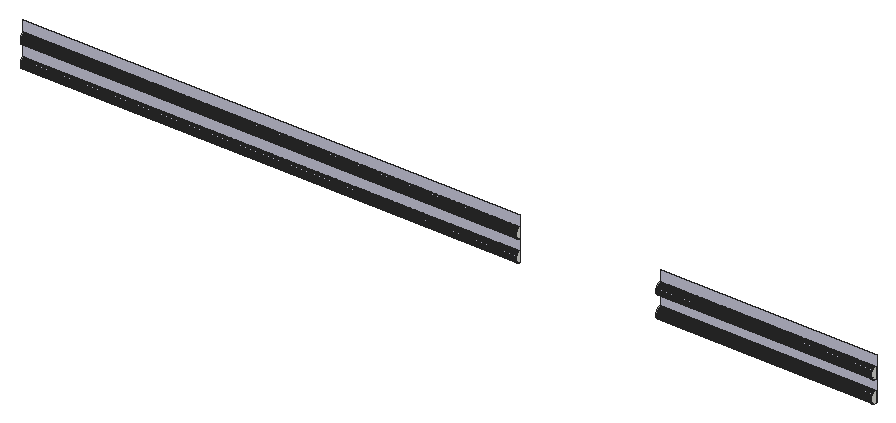
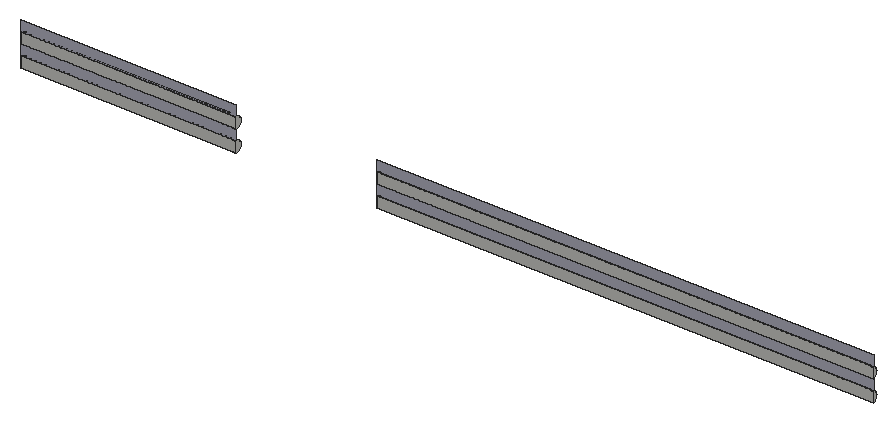
# SketchUp Ruby script. Lengths in millimetres.
U = 1.mm
M = Sketchup.active_model
def pt(a) = Geom::Point3d.new(a.map { |v| v * U })
def face(e, loops, mat)
  f = e.add_face(loops[0].map { |a| pt(a) })
  loops[1..].each { |l| e.add_face(l.map { |a| pt(a) }).erase! }
  f.material = f.back_material = mat if mat
  f
end
# faces: each face lists its corners as indices into pts; further lists are holes
def faces(e, pts, list, mat = nil) = list.each { |f| face(e, (f[0].is_a?(Array) ? f : [f]).map { |l| l.map { |i| pts[i] } }, mat) }
# xy, xz, yz: faces in a plane at the given z, y or x. An outline is a flat list of corners, or four numbers for a rectangle; further outlines are holes
def ring(l) = l.size == 4 ? [[l[0], l[1]], [l[2], l[1]], [l[2], l[3]], [l[0], l[3]]] : l.each_slice(2).to_a
def flat(e, list, mat, &to3) = list.each { |f| face(e, (f[0].is_a?(Array) ? f : [f]).map { |l| ring(l).map { |u, v| to3.(u, v) } }, mat) }
def xy(e, z, list, mat = nil) = flat(e, list, mat) { |x, y| [x, y, z] }
def xz(e, y, list, mat = nil) = flat(e, list, mat) { |x, z| [x, y, z] }
def yz(e, x, list, mat = nil) = flat(e, list, mat) { |y, z| [x, y, z] }
def lines(e, pts, list) = list.each { |a, b| e.add_line(pt(pts[a]), pt(pts[b])) }
# prism: a flat outline (further loops are holes) pulled along v
def prism(e, loops, v, mat = nil)
  f = face(e, loops, mat); d = Geom::Vector3d.new(v.map { |x| x * U })
  f.pushpull(f.normal.samedirection?(d) ? d.length : -d.length)
end
def box(e, o, s, mat = nil) = prism(e, [[o, [o[0] + s[0], o[1], o[2]], [o[0] + s[0], o[1] + s[1], o[2]], [o[0], o[1] + s[1], o[2]]]], [0, 0, s[2]], mat)
def at(x, y, z, deg = 0) = Geom::Transformation.translation(pt([x, y, z])) * Geom::Transformation.rotation(ORIGIN, Z_AXIS, deg.degrees)
def axes(o, x, y, z) = Geom::Transformation.new([*x, 0, *y, 0, *z, 0, *pt(o).to_a, 1])
def part(name) = M.definitions.add(name)
# library, detail: a bought-in or finely detailed component or shape, given as its bounding box
def library(name, o, s) = part(name).tap { |d| box(d.entities, o, s) }
def detail(e, o, s) = box(e.add_group.entities, o, s)
def put(e, d, t, mat = nil) = e.add_instance(d, t).tap { |i| i.material = mat if mat }
def group(e, t, mat = nil) = e.add_group.tap { |g| g.transformation = t; g.material = mat if mat }.entities
root = M.entities
M.materials.add("[0116_Lavender]").color = [197, 197, 214]
xz(root,16548.1,[[11038.5,3825.9,25059.3,4130.7],[29021.7,3825.9,35117.7,4130.7],[11038.5,4435.5,25059.3,4740.3],[29021.7,4435.5,35117.7,4740.3]])
xz(root,16548.1,[[11038.5,4130.7,25059.3,4435.5],[29021.7,4130.7,35117.7,4435.5],[11038.5,4740.3,25059.3,5045.1],[29021.7,4740.3,35117.7,5045.1]],"[0116_Lavender]")
yz(root,11038.5,[[16548.1,3825.9,16536.2,3831.2,16524.8,3837.5,16514,3844.6,16503.7,3852.6,16494.1,3861.4,16485.2,3870.9,16477.1,3881,16469.8,3891.8,16463.4,3903.1,16458,3914.9,16453.4,3927.1,16449.9,3939.6,16447.3,3952.4,16445.8,3965.3,16445.3,3978.3,16445.8,3991.3,16447.3,4004.2,16449.9,4016.9,16453.4,4029.4,16458,4041.6,16463.4,4053.4,16469.8,4064.7,16477.1,4075.5,16485.2,4085.7,16494.1,4095.2,16503.7,4104,16514,4111.9,16524.8,4119.1,16536.2,4125.3,16548.1,4130.7],[16548.1,4435.5,16536.2,4440.8,16524.8,4447.1,16514,4454.2,16503.7,4462.2,16494.1,4471,16485.2,4480.5,16477.1,4490.6,16469.8,4501.4,16463.4,4512.7,16458,4524.5,16453.4,4536.7,16449.9,4549.2,16447.3,4562,16445.8,4574.9,16445.3,4587.9,16445.8,4600.9,16447.3,4613.8,16449.9,4626.5,16453.4,4639,16458,4651.2,16463.4,4663,16469.8,4674.3,16477.1,4685.1,16485.2,4695.3,16494.1,4704.8,16503.7,4713.6,16514,4721.5,16524.8,4728.7,16536.2,4734.9,16548.1,4740.3]])
yz(root,25059.3,[[16548.1,3825.9,16548.1,4130.7,16536.2,4125.3,16524.8,4119.1,16514,4111.9,16503.7,4104,16494.1,4095.2,16485.2,4085.7,16477.1,4075.5,16469.8,4064.7,16463.4,4053.4,16458,4041.6,16453.4,4029.4,16449.9,4016.9,16447.3,4004.2,16445.8,3991.3,16445.3,3978.3,16445.8,3965.3,16447.3,3952.4,16449.9,3939.6,16453.4,3927.1,16458,3914.9,16463.4,3903.1,16469.8,3891.8,16477.1,3881,16485.2,3870.9,16494.1,3861.4,16503.7,3852.6,16514,3844.6,16524.8,3837.5,16536.2,3831.2],[16548.1,4435.5,16548.1,4740.3,16536.2,4734.9,16524.8,4728.7,16514,4721.5,16503.7,4713.6,16494.1,4704.8,16485.2,4695.3,16477.1,4685.1,16469.8,4674.3,16463.4,4663,16458,4651.2,16453.4,4639,16449.9,4626.5,16447.3,4613.8,16445.8,4600.9,16445.3,4587.9,16445.8,4574.9,16447.3,4562,16449.9,4549.2,16453.4,4536.7,16458,4524.5,16463.4,4512.7,16469.8,4501.4,16477.1,4490.6,16485.2,4480.5,16494.1,4471,16503.7,4462.2,16514,4454.2,16524.8,4447.1,16536.2,4440.8]])
yz(root,29021.7,[[16548.1,3825.9,16540.1,3826.1,16532.2,3826.7,16524.3,3827.8,16516.4,3829.2,16508.7,3831.1,16501,3833.3,16493.5,3836,16486.1,3839.1,16478.9,3842.5,16471.9,3846.3,16465.1,3850.5,16458.5,3855,16452.2,3859.8,16446.1,3865,16440.3,3870.5,16434.8,3876.3,16429.7,3882.4,16424.8,3888.7,16420.3,3895.3,16416.1,3902.1,16412.3,3909.1,16408.9,3916.3,16405.8,3923.7,16403.2,3931.2,16400.9,3938.8,16399,3946.6,16397.6,3954.4,16396.5,3962.3,16395.9,3970.3,16395.7,3978.3,16395.9,3986.3,16396.5,3994.2,16397.6,4002.1,16399,4010,16400.9,4017.7,16403.2,4025.4,16405.8,4032.9,16408.9,4040.3,16412.3,4047.5,16416.1,4054.5,16420.3,4061.3,16424.8,4067.9,16429.7,4074.2,16434.8,4080.3,16440.3,4086,16446.1,4091.5,16452.2,4096.7,16458.5,4101.6,16465.1,4106.1,16471.9,4110.3,16478.9,4114.1,16486.1,4117.5,16493.5,4120.6,16501,4123.2,16508.7,4125.5,16516.4,4127.3,16524.3,4128.8,16532.2,4129.8,16540.1,4130.5,16548.1,4130.7],[16548.1,4435.5,16540.1,4435.7,16532.2,4436.3,16524.3,4437.4,16516.4,4438.8,16508.7,4440.7,16501,4442.9,16493.5,4445.6,16486.1,4448.7,16478.9,4452.1,16471.9,4455.9,16465.1,4460.1,16458.5,4464.6,16452.2,4469.4,16446.1,4474.6,16440.3,4480.1,16434.8,4485.9,16429.7,4492,16424.8,4498.3,16420.3,4504.9,16416.1,4511.7,16412.3,4518.7,16408.9,4525.9,16405.8,4533.3,16403.2,4540.8,16400.9,4548.4,16399,4556.2,16397.6,4564,16396.5,4571.9,16395.9,4579.9,16395.7,4587.9,16395.9,4595.9,16396.5,4603.8,16397.6,4611.7,16399,4619.6,16400.9,4627.3,16403.2,4635,16405.8,4642.5,16408.9,4649.9,16412.3,4657.1,16416.1,4664.1,16420.3,4670.9,16424.8,4677.5,16429.7,4683.8,16434.8,4689.9,16440.3,4695.6,16446.1,4701.1,16452.2,4706.3,16458.5,4711.2,16465.1,4715.7,16471.9,4719.9,16478.9,4723.7,16486.1,4727.1,16493.5,4730.2,16501,4732.8,16508.7,4735.1,16516.4,4736.9,16524.3,4738.4,16532.2,4739.4,16540.1,4740.1,16548.1,4740.3]])
yz(root,35117.7,[[16548.1,3825.9,16548.1,4130.7,16540.1,4130.5,16532.2,4129.8,16524.3,4128.8,16516.4,4127.3,16508.7,4125.5,16501,4123.2,16493.5,4120.6,16486.1,4117.5,16478.9,4114.1,16471.9,4110.3,16465.1,4106.1,16458.5,4101.6,16452.2,4096.7,16446.1,4091.5,16440.3,4086,16434.8,4080.3,16429.7,4074.2,16424.8,4067.9,16420.3,4061.3,16416.1,4054.5,16412.3,4047.5,16408.9,4040.3,16405.8,4032.9,16403.2,4025.4,16400.9,4017.7,16399,4010,16397.6,4002.1,16396.5,3994.2,16395.9,3986.3,16395.7,3978.3,16395.9,3970.3,16396.5,3962.3,16397.6,3954.4,16399,3946.6,16400.9,3938.8,16403.2,3931.2,16405.8,3923.7,16408.9,3916.3,16412.3,3909.1,16416.1,3902.1,16420.3,3895.3,16424.8,3888.7,16429.7,3882.4,16434.8,3876.3,16440.3,3870.5,16446.1,3865,16452.2,3859.8,16458.5,3855,16465.1,3850.5,16471.9,3846.3,16478.9,3842.5,16486.1,3839.1,16493.5,3836,16501,3833.3,16508.7,3831.1,16516.4,3829.2,16524.3,3827.8,16532.2,3826.7,16540.1,3826.1],[16548.1,4435.5,16548.1,4740.3,16540.1,4740.1,16532.2,4739.4,16524.3,4738.4,16516.4,4736.9,16508.7,4735.1,16501,4732.8,16493.5,4730.2,16486.1,4727.1,16478.9,4723.7,16471.9,4719.9,16465.1,4715.7,16458.5,4711.2,16452.2,4706.3,16446.1,4701.1,16440.3,4695.6,16434.8,4689.9,16429.7,4683.8,16424.8,4677.5,16420.3,4670.9,16416.1,4664.1,16412.3,4657.1,16408.9,4649.9,16405.8,4642.5,16403.2,4635,16400.9,4627.3,16399,4619.6,16397.6,4611.7,16396.5,4603.8,16395.9,4595.9,16395.7,4587.9,16395.9,4579.9,16396.5,4571.9,16397.6,4564,16399,4556.2,16400.9,4548.4,16403.2,4540.8,16405.8,4533.3,16408.9,4525.9,16412.3,4518.7,16416.1,4511.7,16420.3,4504.9,16424.8,4498.3,16429.7,4492,16434.8,4485.9,16440.3,4480.1,16446.1,4474.6,16452.2,4469.4,16458.5,4464.6,16465.1,4460.1,16471.9,4455.9,16478.9,4452.1,16486.1,4448.7,16493.5,4445.6,16501,4442.9,16508.7,4440.7,16516.4,4438.8,16524.3,4437.4,16532.2,4436.3,16540.1,4435.7]])
p = [[25059.3,16548.1,3825.9],[25059.3,16536.2,3831.2],[11038.5,16536.2,3831.2],[11038.5,16548.1,3825.9],[35117.7,16548.1,3825.9],[35117.7,16540.1,3826.1],
  [29021.7,16540.1,3826.1],[29021.7,16548.1,3825.9],[35117.7,16532.2,3826.7],[29021.7,16532.2,3826.7],[35117.7,16524.3,3827.8],[29021.7,16524.3,3827.8],
  [35117.7,16516.4,3829.2],[29021.7,16516.4,3829.2],[35117.7,16508.7,3831.1],[29021.7,16508.7,3831.1],[35117.7,16501,3833.3],[29021.7,16501,3833.3],
  [25059.3,16524.8,3837.5],[11038.5,16524.8,3837.5],[35117.7,16493.5,3836],[29021.7,16493.5,3836],[35117.7,16486.1,3839.1],[29021.7,16486.1,3839.1],
  [25059.3,16514,3844.6],[11038.5,16514,3844.6],[35117.7,16478.9,3842.5],[29021.7,16478.9,3842.5],[35117.7,16471.9,3846.3],[29021.7,16471.9,3846.3],
  [25059.3,16503.7,3852.6],[11038.5,16503.7,3852.6],[35117.7,16465.1,3850.5],[29021.7,16465.1,3850.5],[35117.7,16458.5,3855],[29021.7,16458.5,3855],
  [25059.3,16494.1,3861.4],[11038.5,16494.1,3861.4],[35117.7,16452.2,3859.8],[29021.7,16452.2,3859.8],[35117.7,16446.1,3865],[29021.7,16446.1,3865],
  [25059.3,16485.2,3870.9],[11038.5,16485.2,3870.9],[35117.7,16440.3,3870.5],[29021.7,16440.3,3870.5],[35117.7,16434.8,3876.3],[29021.7,16434.8,3876.3],
  [25059.3,16477.1,3881],[11038.5,16477.1,3881],[35117.7,16429.7,3882.4],[29021.7,16429.7,3882.4],[25059.3,16469.8,3891.8],[11038.5,16469.8,3891.8],
  [35117.7,16424.8,3888.7],[29021.7,16424.8,3888.7],[35117.7,16420.3,3895.3],[29021.7,16420.3,3895.3],[25059.3,16463.4,3903.1],[11038.5,16463.4,3903.1],
  [35117.7,16416.1,3902.1],[29021.7,16416.1,3902.1],[35117.7,16412.3,3909.1],[29021.7,16412.3,3909.1],[25059.3,16458,3914.9],[11038.5,16458,3914.9],
  [35117.7,16408.9,3916.3],[29021.7,16408.9,3916.3],[25059.3,16453.4,3927.1],[11038.5,16453.4,3927.1],[35117.7,16405.8,3923.7],[29021.7,16405.8,3923.7],
  [35117.7,16403.2,3931.2],[29021.7,16403.2,3931.2],[25059.3,16449.9,3939.6],[11038.5,16449.9,3939.6],[35117.7,16400.9,3938.8],[29021.7,16400.9,3938.8],
  [35117.7,16399,3946.6],[29021.7,16399,3946.6],[25059.3,16447.3,3952.4],[11038.5,16447.3,3952.4],[35117.7,16397.6,3954.4],[29021.7,16397.6,3954.4],
  [25059.3,16445.8,3965.3],[11038.5,16445.8,3965.3],[35117.7,16396.5,3962.3],[29021.7,16396.5,3962.3],[35117.7,16395.9,3970.3],[29021.7,16395.9,3970.3],
  [25059.3,16445.3,3978.3],[11038.5,16445.3,3978.3],[35117.7,16395.7,3978.3],[29021.7,16395.7,3978.3],[35117.7,16395.9,3986.3],[29021.7,16395.9,3986.3],
  [25059.3,16445.8,3991.3],[11038.5,16445.8,3991.3],[35117.7,16396.5,3994.2],[29021.7,16396.5,3994.2],[25059.3,16447.3,4004.2],[11038.5,16447.3,4004.2],
  [35117.7,16397.6,4002.1],[29021.7,16397.6,4002.1],[35117.7,16399,4010],[29021.7,16399,4010],[25059.3,16449.9,4016.9],[11038.5,16449.9,4016.9],
  [35117.7,16400.9,4017.7],[29021.7,16400.9,4017.7],[25059.3,16453.4,4029.4],[11038.5,16453.4,4029.4],[35117.7,16403.2,4025.4],[29021.7,16403.2,4025.4],
  [35117.7,16405.8,4032.9],[29021.7,16405.8,4032.9],[25059.3,16458,4041.6],[11038.5,16458,4041.6],[35117.7,16408.9,4040.3],[29021.7,16408.9,4040.3],
  [35117.7,16412.3,4047.5],[29021.7,16412.3,4047.5],[25059.3,16463.4,4053.4],[11038.5,16463.4,4053.4],[35117.7,16416.1,4054.5],[29021.7,16416.1,4054.5],
  [25059.3,16469.8,4064.7],[11038.5,16469.8,4064.7],[35117.7,16420.3,4061.3],[29021.7,16420.3,4061.3],[35117.7,16424.8,4067.9],[29021.7,16424.8,4067.9],
  [25059.3,16477.1,4075.5],[11038.5,16477.1,4075.5],[35117.7,16429.7,4074.2],[29021.7,16429.7,4074.2],[35117.7,16434.8,4080.3],[29021.7,16434.8,4080.3],
  [25059.3,16485.2,4085.7],[11038.5,16485.2,4085.7],[35117.7,16440.3,4086],[29021.7,16440.3,4086],[25059.3,16494.1,4095.2],[11038.5,16494.1,4095.2],
  [35117.7,16446.1,4091.5],[29021.7,16446.1,4091.5],[35117.7,16452.2,4096.7],[29021.7,16452.2,4096.7],[25059.3,16503.7,4104],[11038.5,16503.7,4104],
  [35117.7,16458.5,4101.6],[29021.7,16458.5,4101.6],[35117.7,16465.1,4106.1],[29021.7,16465.1,4106.1],[25059.3,16514,4111.9],[11038.5,16514,4111.9],
  [35117.7,16471.9,4110.3],[29021.7,16471.9,4110.3],[35117.7,16478.9,4114.1],[29021.7,16478.9,4114.1],[25059.3,16524.8,4119.1],[11038.5,16524.8,4119.1],
  [35117.7,16486.1,4117.5],[29021.7,16486.1,4117.5],[35117.7,16493.5,4120.6],[29021.7,16493.5,4120.6],[25059.3,16536.2,4125.3],[11038.5,16536.2,4125.3],
  [35117.7,16501,4123.2],[29021.7,16501,4123.2],[35117.7,16508.7,4125.5],[29021.7,16508.7,4125.5],[25059.3,16548.1,4130.7],[11038.5,16548.1,4130.7],
  [35117.7,16516.4,4127.3],[29021.7,16516.4,4127.3],[35117.7,16524.3,4128.8],[29021.7,16524.3,4128.8],[35117.7,16532.2,4129.8],[29021.7,16532.2,4129.8],
  [35117.7,16540.1,4130.5],[29021.7,16540.1,4130.5],[35117.7,16548.1,4130.7],[29021.7,16548.1,4130.7],[25059.3,16548.1,4435.5],[25059.3,16536.2,4440.8],
  [11038.5,16536.2,4440.8],[11038.5,16548.1,4435.5],[35117.7,16548.1,4435.5],[35117.7,16540.1,4435.7],[29021.7,16540.1,4435.7],[29021.7,16548.1,4435.5],
  [35117.7,16532.2,4436.3],[29021.7,16532.2,4436.3],[35117.7,16524.3,4437.4],[29021.7,16524.3,4437.4],[35117.7,16516.4,4438.8],[29021.7,16516.4,4438.8],
  [35117.7,16508.7,4440.7],[29021.7,16508.7,4440.7],[35117.7,16501,4442.9],[29021.7,16501,4442.9],[25059.3,16524.8,4447.1],[11038.5,16524.8,4447.1],
  [35117.7,16493.5,4445.6],[29021.7,16493.5,4445.6],[35117.7,16486.1,4448.7],[29021.7,16486.1,4448.7],[25059.3,16514,4454.2],[11038.5,16514,4454.2],
  [35117.7,16478.9,4452.1],[29021.7,16478.9,4452.1],[35117.7,16471.9,4455.9],[29021.7,16471.9,4455.9],[25059.3,16503.7,4462.2],[11038.5,16503.7,4462.2],
  [35117.7,16465.1,4460.1],[29021.7,16465.1,4460.1],[35117.7,16458.5,4464.6],[29021.7,16458.5,4464.6],[25059.3,16494.1,4471],[11038.5,16494.1,4471],
  [35117.7,16452.2,4469.4],[29021.7,16452.2,4469.4],[35117.7,16446.1,4474.6],[29021.7,16446.1,4474.6],[25059.3,16485.2,4480.5],[11038.5,16485.2,4480.5],
  [35117.7,16440.3,4480.1],[29021.7,16440.3,4480.1],[35117.7,16434.8,4485.9],[29021.7,16434.8,4485.9],[25059.3,16477.1,4490.6],[11038.5,16477.1,4490.6],
  [35117.7,16429.7,4492],[29021.7,16429.7,4492],[25059.3,16469.8,4501.4],[11038.5,16469.8,4501.4],[35117.7,16424.8,4498.3],[29021.7,16424.8,4498.3],
  [35117.7,16420.3,4504.9],[29021.7,16420.3,4504.9],[25059.3,16463.4,4512.7],[11038.5,16463.4,4512.7],[35117.7,16416.1,4511.7],[29021.7,16416.1,4511.7],
  [35117.7,16412.3,4518.7],[29021.7,16412.3,4518.7],[25059.3,16458,4524.5],[11038.5,16458,4524.5],[35117.7,16408.9,4525.9],[29021.7,16408.9,4525.9],
  [25059.3,16453.4,4536.7],[11038.5,16453.4,4536.7],[35117.7,16405.8,4533.3],[29021.7,16405.8,4533.3],[35117.7,16403.2,4540.8],[29021.7,16403.2,4540.8],
  [25059.3,16449.9,4549.2],[11038.5,16449.9,4549.2],[35117.7,16400.9,4548.4],[29021.7,16400.9,4548.4],[35117.7,16399,4556.2],[29021.7,16399,4556.2],
  [25059.3,16447.3,4562],[11038.5,16447.3,4562],[35117.7,16397.6,4564],[29021.7,16397.6,4564],[25059.3,16445.8,4574.9],[11038.5,16445.8,4574.9],
  [35117.7,16396.5,4571.9],[29021.7,16396.5,4571.9],[35117.7,16395.9,4579.9],[29021.7,16395.9,4579.9],[25059.3,16445.3,4587.9],[11038.5,16445.3,4587.9],
  [35117.7,16395.7,4587.9],[29021.7,16395.7,4587.9],[35117.7,16395.9,4595.9],[29021.7,16395.9,4595.9],[25059.3,16445.8,4600.9],[11038.5,16445.8,4600.9],
  [35117.7,16396.5,4603.8],[29021.7,16396.5,4603.8],[25059.3,16447.3,4613.8],[11038.5,16447.3,4613.8],[35117.7,16397.6,4611.7],[29021.7,16397.6,4611.7],
  [35117.7,16399,4619.6],[29021.7,16399,4619.6],[25059.3,16449.9,4626.5],[11038.5,16449.9,4626.5],[35117.7,16400.9,4627.3],[29021.7,16400.9,4627.3],
  [25059.3,16453.4,4639],[11038.5,16453.4,4639],[35117.7,16403.2,4635],[29021.7,16403.2,4635],[35117.7,16405.8,4642.5],[29021.7,16405.8,4642.5],
  [25059.3,16458,4651.2],[11038.5,16458,4651.2],[35117.7,16408.9,4649.9],[29021.7,16408.9,4649.9],[35117.7,16412.3,4657.1],[29021.7,16412.3,4657.1],
  [25059.3,16463.4,4663],[11038.5,16463.4,4663],[35117.7,16416.1,4664.1],[29021.7,16416.1,4664.1],[25059.3,16469.8,4674.3],[11038.5,16469.8,4674.3],
  [35117.7,16420.3,4670.9],[29021.7,16420.3,4670.9],[35117.7,16424.8,4677.5],[29021.7,16424.8,4677.5],[25059.3,16477.1,4685.1],[11038.5,16477.1,4685.1],
  [35117.7,16429.7,4683.8],[29021.7,16429.7,4683.8],[35117.7,16434.8,4689.9],[29021.7,16434.8,4689.9],[25059.3,16485.2,4695.3],[11038.5,16485.2,4695.3],
  [35117.7,16440.3,4695.6],[29021.7,16440.3,4695.6],[25059.3,16494.1,4704.8],[11038.5,16494.1,4704.8],[35117.7,16446.1,4701.1],[29021.7,16446.1,4701.1],
  [35117.7,16452.2,4706.3],[29021.7,16452.2,4706.3],[25059.3,16503.7,4713.6],[11038.5,16503.7,4713.6],[35117.7,16458.5,4711.2],[29021.7,16458.5,4711.2],
  [35117.7,16465.1,4715.7],[29021.7,16465.1,4715.7],[25059.3,16514,4721.5],[11038.5,16514,4721.5],[35117.7,16471.9,4719.9],[29021.7,16471.9,4719.9],
  [35117.7,16478.9,4723.7],[29021.7,16478.9,4723.7],[25059.3,16524.8,4728.7],[11038.5,16524.8,4728.7],[35117.7,16486.1,4727.1],[29021.7,16486.1,4727.1],
  [35117.7,16493.5,4730.2],[29021.7,16493.5,4730.2],[25059.3,16536.2,4734.9],[11038.5,16536.2,4734.9],[35117.7,16501,4732.8],[29021.7,16501,4732.8],
  [35117.7,16508.7,4735.1],[29021.7,16508.7,4735.1],[25059.3,16548.1,4740.3],[11038.5,16548.1,4740.3],[35117.7,16516.4,4736.9],[29021.7,16516.4,4736.9],
  [35117.7,16524.3,4738.4],[29021.7,16524.3,4738.4],[35117.7,16532.2,4739.4],[29021.7,16532.2,4739.4],[35117.7,16540.1,4740.1],[29021.7,16540.1,4740.1],
  [35117.7,16548.1,4740.3],[29021.7,16548.1,4740.3]]
faces(root,p,[[0,1,2,3],[4,5,6,7],[5,8,9,6],[8,10,11,9],[10,12,13,11],[12,14,15,13],[14,16,17,15],[1,18,19,2],
  [16,20,21,17],[20,22,23,21],[18,24,25,19],[22,26,27,23],[26,28,29,27],[24,30,31,25],[28,32,33,29],[32,34,35,33],
  [30,36,37,31],[34,38,39,35],[38,40,41,39],[36,42,43,37],[40,44,45,41],[44,46,47,45],[42,48,49,43],[46,50,51,47],
  [48,52,53,49],[50,54,55,51],[54,56,57,55],[52,58,59,53],[56,60,61,57],[60,62,63,61],[58,64,65,59],[62,66,67,63],
  [64,68,69,65],[66,70,71,67],[70,72,73,71],[68,74,75,69],[72,76,77,73],[76,78,79,77],[74,80,81,75],[78,82,83,79],
  [80,84,85,81],[82,86,87,83],[86,88,89,87],[84,90,91,85],[88,92,93,89],[92,94,95,93],[90,96,97,91],[94,98,99,95],
  [96,100,101,97],[98,102,103,99],[102,104,105,103],[100,106,107,101],[104,108,109,105],[106,110,111,107],[108,112,113,109],[112,114,115,113],
  [110,116,117,111],[114,118,119,115],[118,120,121,119],[116,122,123,117],[120,124,125,121],[122,126,127,123],[124,128,129,125],[128,130,131,129],
  [126,132,133,127],[130,134,135,131],[134,136,137,135],[132,138,139,133],[136,140,141,137],[138,142,143,139],[140,144,145,141],[144,146,147,145],
  [142,148,149,143],[146,150,151,147],[150,152,153,151],[148,154,155,149],[152,156,157,153],[156,158,159,157],[154,160,161,155],[158,162,163,159],
  [162,164,165,163],[160,166,167,161],[164,168,169,165],[168,170,171,169],[166,172,173,167],[170,174,175,171],[174,176,177,175],[176,178,179,177],
  [178,180,181,179],[180,182,183,181],[184,185,186,187],[188,189,190,191],[189,192,193,190],[192,194,195,193],[194,196,197,195],[196,198,199,197],
  [198,200,201,199],[185,202,203,186],[200,204,205,201],[204,206,207,205],[202,208,209,203],[206,210,211,207],[210,212,213,211],[208,214,215,209],
  [212,216,217,213],[216,218,219,217],[214,220,221,215],[218,222,223,219],[222,224,225,223],[220,226,227,221],[224,228,229,225],[228,230,231,229],
  [226,232,233,227],[230,234,235,231],[232,236,237,233],[234,238,239,235],[238,240,241,239],[236,242,243,237],[240,244,245,241],[244,246,247,245],
  [242,248,249,243],[246,250,251,247],[248,252,253,249],[250,254,255,251],[254,256,257,255],[252,258,259,253],[256,260,261,257],[260,262,263,261],
  [258,264,265,259],[262,266,267,263],[264,268,269,265],[266,270,271,267],[270,272,273,271],[268,274,275,269],[272,276,277,273],[276,278,279,277],
  [274,280,281,275],[278,282,283,279],[280,284,285,281],[282,286,287,283],[286,288,289,287],[284,290,291,285],[288,292,293,289],[290,294,295,291],
  [292,296,297,293],[296,298,299,297],[294,300,301,295],[298,302,303,299],[302,304,305,303],[300,306,307,301],[304,308,309,305],[306,310,311,307],
  [308,312,313,309],[312,314,315,313],[310,316,317,311],[314,318,319,315],[318,320,321,319],[316,322,323,317],[320,324,325,321],[322,326,327,323],
  [324,328,329,325],[328,330,331,329],[326,332,333,327],[330,334,335,331],[334,336,337,335],[332,338,339,333],[336,340,341,337],[340,342,343,341],
  [338,344,345,339],[342,346,347,343],[346,348,349,347],[344,350,351,345],[348,352,353,349],[352,354,355,353],[350,356,357,351],[354,358,359,355],
  [358,360,361,359],[360,362,363,361],[362,364,365,363],[364,366,367,365]],"[0116_Lavender]")
